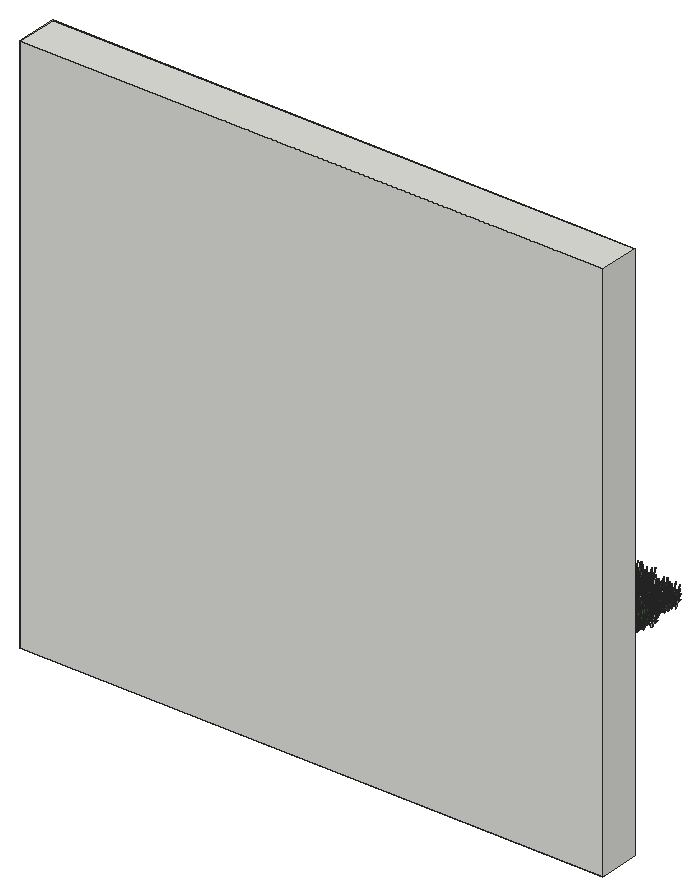
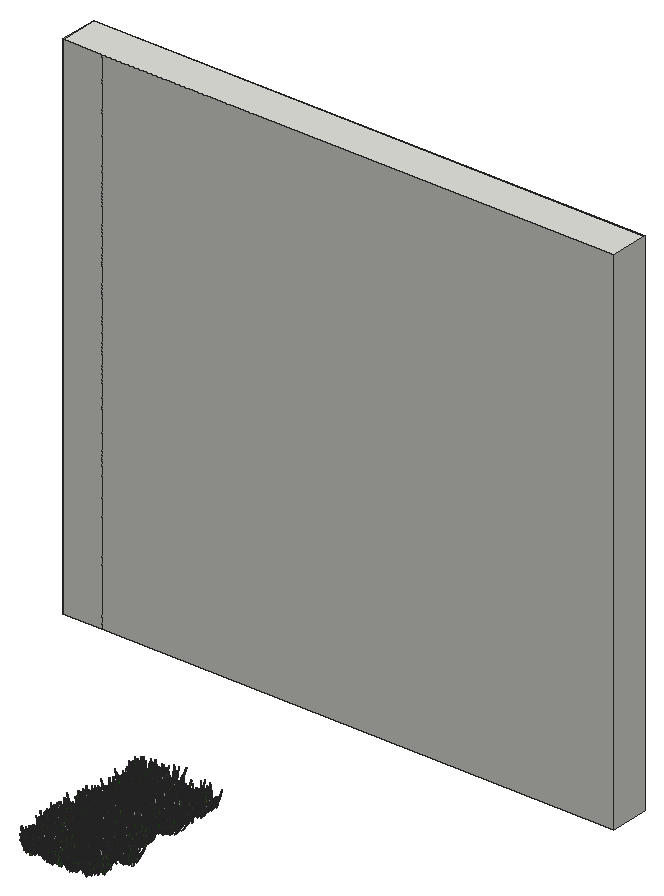
# SketchUp Ruby script. Lengths in inches.
U = 1.inch
M = Sketchup.active_model
def pt(a) = Geom::Point3d.new(a.map { |v| v * U })
def face(e, loops, mat)
  f = e.add_face(loops[0].map { |a| pt(a) })
  loops[1..].each { |l| e.add_face(l.map { |a| pt(a) }).erase! }
  f.material = f.back_material = mat if mat
  f
end
# faces: each face lists its corners as indices into pts; further lists are holes
def faces(e, pts, list, mat = nil) = list.each { |f| face(e, (f[0].is_a?(Array) ? f : [f]).map { |l| l.map { |i| pts[i] } }, mat) }
# xy, xz, yz: faces in a plane at the given z, y or x. An outline is a flat list of corners, or four numbers for a rectangle; further outlines are holes
def ring(l) = l.size == 4 ? [[l[0], l[1]], [l[2], l[1]], [l[2], l[3]], [l[0], l[3]]] : l.each_slice(2).to_a
def flat(e, list, mat, &to3) = list.each { |f| face(e, (f[0].is_a?(Array) ? f : [f]).map { |l| ring(l).map { |u, v| to3.(u, v) } }, mat) }
def xy(e, z, list, mat = nil) = flat(e, list, mat) { |x, y| [x, y, z] }
def xz(e, y, list, mat = nil) = flat(e, list, mat) { |x, z| [x, y, z] }
def yz(e, x, list, mat = nil) = flat(e, list, mat) { |y, z| [x, y, z] }
def lines(e, pts, list) = list.each { |a, b| e.add_line(pt(pts[a]), pt(pts[b])) }
# prism: a flat outline (further loops are holes) pulled along v
def prism(e, loops, v, mat = nil)
  f = face(e, loops, mat); d = Geom::Vector3d.new(v.map { |x| x * U })
  f.pushpull(f.normal.samedirection?(d) ? d.length : -d.length)
end
def box(e, o, s, mat = nil) = prism(e, [[o, [o[0] + s[0], o[1], o[2]], [o[0] + s[0], o[1] + s[1], o[2]], [o[0], o[1] + s[1], o[2]]]], [0, 0, s[2]], mat)
def at(x, y, z, deg = 0) = Geom::Transformation.translation(pt([x, y, z])) * Geom::Transformation.rotation(ORIGIN, Z_AXIS, deg.degrees)
def axes(o, x, y, z) = Geom::Transformation.new([*x, 0, *y, 0, *z, 0, *pt(o).to_a, 1])
def part(name) = M.definitions.add(name)
# library, detail: a bought-in or finely detailed component or shape, given as its bounding box
def library(name, o, s) = part(name).tap { |d| box(d.entities, o, s) }
def detail(e, o, s) = box(e.add_group.entities, o, s)
def put(e, d, t, mat = nil) = e.add_instance(d, t).tap { |i| i.material = mat if mat }
def group(e, t, mat = nil) = e.add_group.tap { |g| g.transformation = t; g.material = mat if mat }.entities
root = M.entities
M.materials.add("Material1").color = [58, 110, 58]
M.materials.add("Material10").color = [48, 100, 38]
M.materials.add("Material3").color = [68, 110, 58]
M.materials.add("Material4").color = [48, 90, 38]
M.materials.add("Material5").color = [68, 110, 48]
M.materials.add("Material6").color = [48, 90, 48]
M.materials.add("Material8").color = [58, 90, 38]
M.materials.add("Material9").color = [68, 100, 58]
c1 = part("grass00")
p = [[-0.6875,0.15,0],[-0.56,0.08,5.52],[-0.04,0.03,2.76],[0.48,-0.02,0],[0.35,-0.02,5.52],[-0.1,-0.14,5.52],
  [-0.12,0.65,8.37],[-0.42,0.65,8.37]]
faces(c1.entities,p,[[0,1,2,3],[3,2,4],[1,5,2],[5,4,2],[1,6,5],[4,5,6],[7,6,1]])
c2 = part("Group16\#1")
put(c2.entities,c1,axes([1.44,-0.61,-0.01],[0.05352,0.12609,0],[-0.10704,0.04543,0.07239],[0.06664,-0.02828,0.11628]),"Material6")
put(c2.entities,c1,axes([0.76,-0.15,-0.01],[0.04676,0.24062,0],[-0.23162,0.04501,0.06642],[0.0652,-0.01267,0.23595]),"Material3")
put(c2.entities,c1,axes([0.79,0.01,-0.01],[-0.00606,0.34651,0],[-0.34381,-0.00602,0.0432],[0.04319,0.00076,0.34386]))
put(c2.entities,c1,axes([1,0.23,-0.01],[-0.07192,0.31144,0],[-0.28722,-0.06632,0.1236],[0.12043,0.02781,0.29478]),"Material5")
put(c2.entities,c1,axes([1.66,0.77,-0.01],[-0.13828,0.29651,0],[-0.21551,-0.1005,0.22471],[0.20365,0.09498,0.23779]),"Material10")
put(c2.entities,c1,axes([0.6875,0.52,-0.01],[-0.18126,0.24051,0],[-0.22746,-0.17142,0.09788],[0.07817,0.05891,0.28481]),"Material5")
put(c2.entities,c1,axes([0.68,0.78,-0.01],[-0.215,0.18688,0],[-0.12385,-0.14248,0.21334],[0.13995,0.16101,0.18878]),"Material3")
put(c2.entities,c1,axes([0.56,1,-0.01],[-0.13756,0.07624,0],[-0.06159,-0.11112,0.0927],[0.04494,0.08108,0.12705]),"Material5")
put(c2.entities,c1,axes([0.2,0.64,-0.01],[-0.23729,0.07254,0],[-0.05711,-0.18681,0.153],[0.04473,0.14632,0.19535]),"Material10")
put(c2.entities,c1,axes([0.0625,0.72,-0.01],[-0.28874,0.02525,0],[-0.02179,-0.24916,0.14647],[0.01276,0.14591,0.25012]),"Material3")
put(c2.entities,c1,axes([-0.08,0.62,-0.01],[-0.34089,-0.04187,0],[0.03255,-0.26504,0.216],[-0.02633,0.21439,0.26703]),"Material10")
put(c2.entities,c1,axes([-0.34,0.98,-0.01],[-0.14314,-0.0493,0],[0.04397,-0.12769,0.06843],[-0.02228,0.0647,0.13505]),"Material10")
put(c2.entities,c1,axes([-0.87,1.45,-0.01],[-0.23488,-0.14114,0],[0.13761,-0.22901,0.06087],[-0.03135,0.05217,0.26717]))
put(c2.entities,c1,axes([-0.72,0.77,-0.01],[-0.14208,-0.13251,0],[0.07209,-0.0773,0.16301],[-0.11118,0.11922,0.1057]),"Material10")
put(c2.entities,c1,axes([-0.62,0.43,-0.01],[-0.14845,-0.21203,0],[0.18654,-0.13061,0.12304],[-0.10079,0.07057,0.22772]),"Material3")
put(c2.entities,c1,axes([-0.68,0.29,-0.01],[-0.13639,-0.32136,0],[0.31723,-0.13464,0.05579],[-0.05136,0.0218,0.34462]),"Material4")
put(c2.entities,c1,axes([-0.64,0.125,-0.01],[-0.0458,-0.23569,0],[0.22124,-0.043,0.08276],[-0.08124,0.01579,0.22538]),"Material1")
put(c2.entities,c1,axes([-1.6,-0.03,-0.01],[0.00576,-0.32897,0],[0.27526,0.00482,0.18018],[-0.18015,-0.00315,0.2753]),"Material5")
put(c2.entities,c1,axes([-1.36,-0.31,-0.01],[0.05718,-0.24765,0],[0.18172,0.04196,0.17267],[-0.16825,-0.03885,0.1865]),"Material10")
put(c2.entities,c1,axes([-1.54,-0.72,-0.01],[0.06537,-0.14017,0],[0.13555,0.06321,0.03939],[-0.0357,-0.01665,0.14956]))
put(c2.entities,c1,axes([-1.19,-0.9,-0.01],[0.09597,-0.12735,0],[0.11214,0.08451,0.07557],[-0.06035,-0.04548,0.14042]),"Material9")
put(c2.entities,c1,axes([-0.47,-0.54,-0.01],[0.11588,-0.10072,0],[0.0618,0.0711,0.12124],[-0.07953,-0.0915,0.0942]))
put(c2.entities,c1,axes([-0.47,-0.84,-0.01],[0.11927,-0.0661,0],[0.06603,0.11913,0.00646],[-0.00313,-0.00565,0.13621]),"Material5")
put(c2.entities,c1,axes([-0.38,-1.24,-0.01],[0.28037,-0.08571,0],[0.0618,0.20215,0.20315],[-0.05939,-0.19428,0.21139]),"Material9")
put(c2.entities,c1,axes([-0.06,-0.66,-0.01],[0.22719,-0.01987,0],[0.01247,0.14255,0.17758],[-0.01547,-0.17691,0.1431]),"Material8")
put(c2.entities,c1,axes([0.11,-0.89,-0.01],[0.14882,0.01828,0],[-0.01058,0.08611,0.12229],[0.01491,-0.12138,0.08676]),"Material6")
put(c2.entities,c1,axes([0.25,-0.72,-0.01],[0.20481,0.07053,0],[-0.06206,0.18022,0.10291],[0.03351,-0.0973,0.1906]),"Material6")
put(c2.entities,c1,axes([0.85,-1.42,-0.01],[0.16481,0.09904,0],[-0.09472,0.15762,0.05616],[0.02893,-0.04814,0.18389]),"Material5")
put(c2.entities,c1,axes([1.01,-1.09,-0.01],[0.21858,0.20385,0],[-0.17495,0.1876,0.15339],[0.10462,-0.11218,0.25652]),"Material10")
put(c2.entities,c1,axes([1.01,-0.71,-0.01],[0.08733,0.12473,0],[-0.06445,0.04512,0.13037],[0.1068,-0.07477,0.07867]),"Material6")
c3 = part("Group15\#1")
put(c3.entities,c2,at(0,0,0))
c4 = part("3darcstudiotree_grass00\#1")
put(c4.entities,c3,at(0,0,0))
put(root,c4,axes([280.14,122.01,0.25],[0.96649,0.69,0],[-0.71558,0.6905,-0.04839],[-0.04247,0.04099,1.47711]))
put(root,c4,axes([280.98,108.43,0.25],[-0.66676,-0.67151,0],[0.72285,-0.49444,-0.03867],[0.0477,-0.03263,1.49724]))
put(root,c4,axes([281.09,99.91,0.25],[-0.806,-0.35525,0],[0.5393,-0.84292,-0.05452],[0.03122,-0.0488,1.404]))
put(root,c4,axes([281.11,97.14,0.25],[0.1532,-1.04407,0],[1.04107,0.10524,-0.0324],[0.04538,0.00459,1.47946]))
put(root,c4,axes([281.3,104.07,0.25],[-0.11859,-0.98397,0],[1.04274,-0.08657,-0.05423],[0.08746,-0.00726,1.69842]))
put(root,c4,axes([281.33,106.17,0.25],[-0.91725,0.50365,0],[-0.56826,-0.71295,-0.03289],[-0.02742,-0.03441,1.55622]))
put(root,c4,axes([281.53,109.2,0.25],[-0.76435,-0.59481,0],[0.61932,-0.54826,-0.04465],[0.05797,-0.05132,1.71883]))
put(root,c4,axes([281.74,100.72,0.25],[-0.61176,-0.56382,0],[0.75936,-0.56761,-0.04825],[0.06504,-0.04861,1.85346]))
put(root,c4,axes([281.89,127.21,0.25],[-0.44538,0.78051,0],[-1.01343,-0.39838,-0.05633],[-0.08545,-0.03359,1.88219]))
put(root,c4,axes([282.54,120.57,0.25],[0.24659,-0.81567,0],[1.24028,0.2583,-0.03647],[0.03753,0.00782,1.35653]))
put(root,c4,axes([282.49,113.52,0.25],[0.32185,-0.85158,0],[0.94359,0.24568,-0.02865],[0.04831,0.01258,1.74795]))
put(root,c4,axes([282.39,104.88,0.25],[0.64389,-0.79793,0],[0.85629,0.47602,-0.05113],[0.06464,0.03594,1.56833]))
put(root,c4,axes([282.72,108.55,0.25],[-0.90263,-0.3415,0],[0.38015,-0.6922,-0.0331],[0.02315,-0.04215,1.54531]))
put(root,c4,axes([282.41,106.7,0.25],[0.73285,0.722,0],[-0.72451,0.50662,-0.04423],[-0.04928,0.03446,1.38013]))
put(root,c4,axes([282.86,114.61,0.25],[-0.198,-0.93495,0],[1.04135,-0.15193,-0.04893],[0.07876,-0.01149,1.72817]))
put(root,c4,axes([282.61,122.33,0.25],[1.14207,-0.102,0],[0.13761,1.06147,-0.03237],[0.00412,0.03176,1.52951]))
put(root,c4,axes([283.03,103.375,0.25],[-1.16606,-0.38849,0],[0.34532,-0.71405,-0.04034],[0.02573,-0.05319,1.58691]))
g1 = group(root,at(186.47,48,0))
prism(g1,[[[151.5,9,0],[160.5,9,0],[160.5,0,0],[32.14,0,0],[32.14,9,0]]],[0,0,120])
put(root,c4,axes([282.7,129.27,0.25],[0.32926,0.73623,0],[-0.88152,0.27159,-0.04291],[-0.06174,0.01902,1.44315]))
put(root,c4,axes([282.91,125.12,0.25],[0.71198,-0.69558,0],[0.87959,0.62024,-0.02612],[0.03242,0.02286,1.8801]))
put(root,c4,axes([282.76,98.67,0.25],[-0.09062,0.98179,0],[-1.0736,-0.06826,-0.03234],[-0.05691,-0.00362,1.90052]))
put(root,c4,axes([282.67,116.89,0.25],[1.06044,0.60949,0],[-0.58603,0.70241,-0.05103],[-0.04763,0.05709,1.6877]))
put(root,c4,axes([283.35,110.84,0.25],[0.39396,-0.77569,0],[0.86907,0.30407,-0.03331],[0.04938,0.01728,1.51731]))
put(root,c4,axes([283.38,126.24,0.25],[0.16763,0.79034,0],[-1.21049,0.17687,-0.06022],[-0.08603,0.01257,1.78296]))
put(root,c4,axes([283.39,111.61,0.25],[0.53853,0.6124,0],[-0.87052,0.52736,-0.05552],[-0.05804,0.03516,1.39481]))
put(root,c4,axes([284.24,112.93,0.25],[-1.23083,0.12452,0],[-0.1215,-0.82732,-0.03065],[-0.0073,-0.04972,1.97713]))
put(root,c4,axes([284.36,124.27,0.25],[-0.86307,-0.26422,0],[0.42976,-0.96707,-0.02933],[0.01407,-0.03166,1.72129]))
put(root,c4,axes([284.12,100.69,0.25],[1.06091,-0.11039,0],[0.1522,1.0077,-0.03701],[0.00751,0.0497,1.99511]))
put(root,c4,axes([284.06,116.32,0.25],[1.09581,0.45799,0],[-0.53398,0.88015,-0.03278],[-0.02339,0.03856,1.8841]))
put(root,c4,axes([284.42,112.27,0.25],[0.45131,-0.77831,0],[1.15874,0.46288,-0.06017],[0.07334,0.0293,1.73941]))
put(root,c4,axes([284.17,122.08,0.25],[0.99888,0.1401,0],[-0.16713,0.82088,-0.04218],[-0.013,0.06385,1.85529]))
put(root,c4,axes([284.58,104.35,0.25],[-0.30186,-0.76108,0],[1.1493,-0.31403,-0.05688],[0.08145,-0.02225,1.82396]))
put(root,c4,axes([284.15,109.83,0.25],[1.15021,0.22516,0],[-0.24972,0.8788,-0.02883],[-0.0112,0.03942,1.84132]))
put(root,c4,axes([284.75,123.19,0.25],[-0.72312,-0.52329,0],[0.69977,-0.66616,-0.03875],[0.0408,-0.03885,1.70607]))
put(root,c4,axes([284.55,108.29,0.25],[0.68383,-0.50222,0],[0.78836,0.7395,-0.04815],[0.0527,0.04943,1.9649]))
put(root,c4,axes([284.48,125.64,0.25],[0.97755,0.3703,0],[-0.38502,0.7002,-0.03533],[-0.0295,0.05366,1.86502]))
put(root,c4,axes([284.8125,119.35,0.25],[-0.12292,0.83093,0],[-1.10355,-0.11246,-0.03564],[-0.05441,-0.00554,1.71014]))
put(root,c4,axes([284.75,118.61,0.25],[0.6999,0.62264,0],[-0.94819,0.73425,-0.03325],[-0.02999,0.02322,1.59934]))
put(root,c4,axes([285.35,116.27,0.25],[0.07977,-1.03792,0],[1.09466,0.05796,-0.05413],[0.06849,0.00363,1.39055]))
put(root,c4,axes([285.41,107.9,0.25],[0.16518,-1.06009,0],[1.27092,0.13643,-0.05291],[0.05462,0.00586,1.33374]))
put(root,c4,axes([285.51,114.64,0.25],[0.73988,-0.77354,0],[1.00505,0.66225,-0.06314],[0.05015,0.03304,1.30132]))
put(root,c4,axes([285.9,129.72,0.25],[-0.53978,-0.75827,0],[1.09521,-0.53709,-0.05519],[0.06778,-0.03324,1.81465]))
put(root,c4,axes([285.54,104.98,0.25],[0.1922,0.82569,0],[-0.98101,0.15731,-0.03785],[-0.05301,0.0085,1.42505]))
put(root,c4,axes([286.08,107,0.25],[-1.10209,-0.52404,0],[0.57256,-0.82953,-0.04075],[0.02735,-0.03962,1.55523]))
put(root,c4,axes([286.09,123.16,0.25],[-0.23218,-0.75967,0],[1.05774,-0.22271,-0.05601],[0.08968,-0.01888,1.80254]))
put(root,c4,axes([286.37,121.05,0.25],[-1.03868,-0.27875,0],[0.37896,-0.97279,-0.04655],[0.01837,-0.04716,1.58019]))
put(root,c4,axes([286.02,100.5625,0.25],[0.98254,-0.25265,0],[0.27656,0.74092,-0.04073],[0.01854,0.04967,1.43775]))
put(root,c4,axes([286.03,99.6,0.25],[0.41986,0.75322,0],[-1.13167,0.43457,-0.03574],[-0.04976,0.01911,1.91331]))
put(root,c4,axes([286.16,124.78,0.25],[1.16546,0.46684,0],[-0.47037,0.80896,-0.05424],[-0.02973,0.05113,1.36476]))
put(root,c4,axes([286.47,111.74,0.25],[0.34768,-0.86387,0],[0.85624,0.2374,-0.03453],[0.0639,0.01772,1.76116]))
put(root,c4,axes([286.92,106.86,0.25],[-1.17297,-0.02067,0],[0.02407,-0.94108,-0.04949],[0.00177,-0.06917,1.9102]))
put(root,c4,axes([287.3,120.81,0.25],[-0.61007,-0.79395,0],[0.95148,-0.50366,-0.04256],[0.04955,-0.02623,1.55835]))
put(root,c4,axes([286.97,127.42,0.25],[0.91396,-0.02464,0],[0.04119,1.05258,-0.05593],[0.0023,0.05867,1.60461]))
put(root,c4,axes([287.07,117.22,0.25],[1.02052,0.55135,0],[-0.53482,0.68197,-0.02904],[-0.02865,0.03654,1.7729]))
put(root,c4,axes([287.17,108.65,0.25],[0.83736,0.33838,0],[-0.55915,0.95321,-0.05845],[-0.03084,0.05257,1.53958]))
put(root,c4,axes([287.625,103.1,0.25],[-1.22566,0.31592,0],[-0.30293,-0.80966,-0.03919],[-0.01931,-0.05162,1.69748]))
put(root,c4,axes([287.47,99.875,0.25],[0.97887,-0.22338,0],[0.25967,0.78389,-0.03828],[0.01628,0.04916,1.57185]))
put(root,c4,axes([287.42,115.04,0.25],[1.01452,0.22805,0],[-0.26327,0.80685,-0.0432],[-0.01701,0.05214,1.51727]))
put(root,c4,axes([287.625,100.98,0.25],[-0.59004,0.75476,0],[-0.98006,-0.52782,-0.05659],[-0.05684,-0.03061,1.39892]))
put(root,c4,axes([287.92,112.15,0.25],[0.76894,-0.45763,0],[0.64505,0.74668,-0.04704],[0.04225,0.0489,1.70604]))
put(root,c4,axes([287.92,109.35,0.25],[1.18056,0.12682,0],[-0.16494,1.05779,-0.04718],[-0.00694,0.0445,1.4726]))
put(root,c4,axes([287.99,102.05,0.25],[0.2316,1.00827,0],[-0.94622,0.14973,-0.03349],[-0.05489,0.00869,1.60736]))
put(root,c4,axes([287.99,105.91,0.25],[1.03219,0.4525,0],[-0.48048,0.75505,-0.05015],[-0.04152,0.06525,1.82381]))
put(root,c4,axes([288.62,106.05,0.25],[0.66048,-0.81262,0],[0.83349,0.46669,-0.04469],[0.06734,0.0377,1.8275]))
put(root,c4,axes([288.92,116.05,0.25],[-0.79781,-0.64301,0],[0.72834,-0.62256,-0.03796],[0.04001,-0.0342,1.58175]))
put(root,c4,axes([288.49,124.47,0.25],[-0.01446,0.75216,0],[-1.24873,-0.01654,-0.04794],[-0.0632,-0.00084,1.64652]))
put(root,c4,axes([288.79,117.9,0.25],[0.43992,-0.87485,0],[0.97647,0.33827,-0.05171],[0.0741,0.02567,1.64301]))
put(root,c4,axes([288.66,126.91,0.25],[0.12832,0.79022,0],[-1.17061,0.13096,-0.05207],[-0.07812,0.00874,1.7882]))
put(root,c4,axes([289.1,102.97,0.25],[-0.8223,-0.75997,0],[0.923,-0.68801,-0.05274],[0.06284,-0.04684,1.98669]))
put(root,c4,axes([288.86,123.09,0.25],[1.11111,0.21953,0],[-0.27842,0.97075,-0.06215],[-0.01955,0.06815,1.63292]))
put(root,c4,axes([289.36,119.46,0.25],[-0.90252,-0.41614,0],[0.59502,-0.889,-0.02959],[0.01936,-0.02892,1.65043]))
put(root,c4,axes([288.92,122.25,0.25],[0.40373,0.79991,0],[-1.04976,0.365,-0.03717],[-0.04874,0.01695,1.61797]))
put(root,c4,axes([288.93,110.84,0.25],[0.79847,0.56552,0],[-0.69028,0.67142,-0.03219],[-0.03713,0.03611,1.88986]))
put(root,c4,axes([289.32,107.31,0.25],[1.12258,-0.30459,0],[0.34364,0.87251,-0.04269],[0.02321,0.05894,1.93529]))
put(root,c4,axes([289.49,104.47,0.25],[0.7553,-0.61251,0],[0.83696,0.71099,-0.03867],[0.0393,0.03338,1.7417]))
put(root,c4,axes([290.03,115.75,0.25],[-1.07836,-0.58735,0],[0.50923,-0.64407,-0.04657],[0.05066,-0.06408,1.84036]))
put(root,c4,axes([289.92,119.61,0.25],[0.69922,-0.64094,0],[0.77633,0.58344,-0.04299],[0.04858,0.03651,1.59659]))
put(root,c4,axes([290.17,97.35,0.25],[-0.83056,-0.81172,0],[0.84588,-0.59626,-0.05304],[0.07118,-0.05018,1.95407]))
put(root,c4,axes([289.98,122.11,0.25],[-0.57712,0.80927,0],[-0.96213,-0.47267,-0.03668],[-0.05591,-0.02747,1.98009]))
put(root,c4,axes([290.04,129.82,0.25],[-0.4755,0.85123,0],[-1.1316,-0.43547,-0.04346],[-0.05893,-0.02268,1.86413]))
put(root,c4,axes([290.375,113.57,0.25],[-1.24305,0.08795,0],[-0.08349,-0.8129,-0.04632],[-0.00759,-0.07395,1.89764]))
put(root,c4,axes([290.38,118.09,0.25],[-0.3366,0.79048,0],[-0.85568,-0.25101,-0.03966],[-0.05713,-0.01676,1.38647]))
put(root,c4,axes([290.51,111.18,0.25],[-0.95842,0.70962,0],[-0.69168,-0.64356,-0.04505],[-0.0402,-0.0374,1.39266]))
put(root,c4,axes([290.77,116.66,0.25],[-0.37206,-0.80051,0],[1.04801,-0.33556,-0.03571],[0.05709,-0.01828,1.92492]))
put(root,c4,axes([290.39,128.52,0.25],[0.53635,0.81697,0],[-0.91633,0.41443,-0.025],[-0.04192,0.01896,1.99255]))
put(root,c4,axes([290.84,112.06,0.25],[-1.12484,0.02949,0],[-0.03445,-0.90524,-0.03959],[-0.00189,-0.04972,1.65212]))
put(root,c4,axes([290.43,106.58,0.25],[0.762,0.81603,0],[-0.98717,0.63503,-0.03267],[-0.04011,0.0258,1.93988]))
put(root,c4,axes([290.47,126.36,0.25],[0.38959,0.87785,0],[-1.14834,0.35109,-0.04046],[-0.04842,0.0148,1.56076]))
put(root,c4,axes([290.5,104.11,0.25],[0.00735,0.80444,0],[-1.27856,0.00805,-0.03677],[-0.03983,0.00025,1.38481]))
put(root,c4,axes([290.98,99.38,0.25],[-1.06799,-0.08228,0],[0.11727,-1.04872,-0.06502],[0.00676,-0.06047,1.42798]))
put(root,c4,axes([291,103.25,0.25],[0.37646,-0.94503,0],[1.15519,0.31701,-0.04027],[0.05381,0.01477,1.71232]))
put(root,c4,axes([291.6,110.66,0.25],[-0.25978,-0.80409,0],[1.2428,-0.2766,-0.04199],[0.05612,-0.01249,1.7807]))
put(root,c4,axes([291.7,114.34,0.25],[-0.702,-0.60475,0],[0.80009,-0.63981,-0.03217],[0.03306,-0.02644,1.58546]))
put(root,c4,axes([291.61,103.15,0.25],[-1.15974,0.17681,0],[-0.23333,-1.05436,-0.05609],[-0.01523,-0.06884,1.94158]))
put(root,c4,axes([291.68,108.77,0.25],[-1.05103,-0.44112,0],[0.40767,-0.66914,-0.0255],[0.02475,-0.04062,1.94297]))
put(root,c4,axes([291.6,129.58,0.25],[-0.88188,0.19198,0],[-0.31522,-0.99749,-0.03948],[-0.01275,-0.04035,1.58152]))
put(root,c4,axes([291.52,101.04,0.25],[0.03817,0.87199,0],[-0.96597,0.02913,-0.04285],[-0.08096,0.00244,1.82733]))
put(root,c4,axes([291.57,123.71,0.25],[0.92789,-0.22475,0],[0.34756,0.98849,-0.04654],[0.01412,0.04015,1.34343]))
put(root,c4,axes([291.5,128.36,0.25],[0.99429,0.37074,0],[-0.40917,0.75597,-0.04301],[-0.02965,0.05478,1.6797]))
put(root,c4,axes([291.66,109.25,0.25],[0.96625,-0.29228,0],[0.40926,0.93206,-0.06136],[0.03176,0.07234,1.80687]))
put(root,c4,axes([292.2,99.92,0.25],[-1.17693,0.29826,0],[-0.36809,-1.0006,-0.03433],[-0.01076,-0.02926,1.35329]))
put(root,c4,axes([292.15,105.75,0.25],[-0.17663,0.73999,0],[-1.12217,-0.18452,-0.03573],[-0.05134,-0.00844,1.67549]))
put(root,c4,axes([292.33,111.77,0.25],[-0.24663,0.96758,0],[-1.21778,-0.21384,-0.05558],[-0.06952,-0.01221,1.59125]))
put(root,c4,axes([293,108.58,0.25],[-0.43903,-0.74591,0],[0.90583,-0.36729,-0.0349],[0.05733,-0.02325,1.84302]))
put(root,c4,axes([293.16,116.25,0.25],[-1.05707,-0.00531,0],[0.00764,-1.04694,-0.0591],[0.00043,-0.05923,1.52309]))
put(root,c4,axes([293.22,113.8,0.25],[-1.17737,-0.08134,0],[0.09201,-0.91752,-0.036],[0.00525,-0.05238,1.9513]))
put(root,c4,axes([293.1,120.42,0.25],[0.22942,-0.80247,0],[0.87812,0.17294,-0.04624],[0.09726,0.01916,1.95114]))
put(root,c4,axes([293.1,126.04,0.25],[-0.55637,0.80922,0],[-0.80968,-0.3835,-0.04437],[-0.06055,-0.02868,1.46464]))
put(root,c4,axes([293.35,97.26,0.25],[0.33509,-0.89072,0],[1.18941,0.30825,-0.04262],[0.0593,0.01537,1.81655]))
put(root,c4,axes([293.36,104.52,0.25],[-0.67254,0.91689,0],[-0.85898,-0.43406,-0.03488],[-0.04061,-0.02052,1.37068]))
put(root,c4,axes([293.24,107.32,0.25],[0.92619,-0.10185,0],[0.12918,0.80925,-0.04905],[0.00971,0.06081,1.48186]))
put(root,c4,axes([293.41,99.89,0.25],[0.87821,-0.27516,0],[0.35278,0.77567,-0.04981],[0.0297,0.06529,1.68613]))
put(root,c4,axes([293.75,114.91,0.25],[-0.56452,-0.83255,0],[0.9394,-0.43881,-0.05229],[0.06965,-0.03253,1.64764]))
put(root,c4,axes([293.53,109.625,0.25],[-0.60052,0.95546,0],[-1.10338,-0.47774,-0.04188],[-0.0563,-0.02437,1.88687]))
put(root,c4,axes([293.36,122.25,0.25],[0.78993,0.53505,0],[-0.70019,0.71214,-0.03119],[-0.03391,0.03449,1.90467]))
put(root,c4,axes([293.67,128.55,0.25],[-0.50113,0.91608,0],[-0.83688,-0.31538,-0.0444],[-0.07161,-0.02699,1.62807]))
put(root,c4,axes([293.77,118.05,0.25],[-0.62087,0.78586,0],[-1.03493,-0.56328,-0.05216],[-0.04615,-0.02512,1.30947]))
put(root,c4,axes([293.77,119.28,0.25],[-0.50471,0.92883,0],[-1.16901,-0.43761,-0.03185],[-0.04122,-0.01543,1.82087]))
put(root,c4,axes([293.79,103.3,0.25],[0.56865,0.58347,0],[-0.72151,0.48442,-0.02717],[-0.04145,0.02783,1.82093]))
put(root,c4,axes([293.82,98.21,0.25],[0.94731,0.21958,0],[-0.24315,0.72265,-0.03829],[-0.01599,0.04753,1.40372]))
put(root,c4,axes([293.96,124.92,0.25],[1.08833,-0.17129,0],[0.24008,1.05081,-0.05959],[0.01345,0.05887,1.56123]))
put(root,c4,axes([294.57,98.01,0.25],[-0.98856,-0.22721,0],[0.32875,-0.98537,-0.02644],[0.01092,-0.03274,1.9068]))
put(root,c4,axes([294.76,121,0.25],[-1.06378,-0.45854,0],[0.55437,-0.88599,-0.03725],[0.0222,-0.03547,1.55507]))
put(root,c4,axes([294.55,128.33,0.25],[-0.74093,0.83806,0],[-0.99545,-0.60629,-0.06171],[-0.06944,-0.04229,1.72322]))
put(root,c4,axes([294.48,124.32,0.25],[0.46742,0.64787,0],[-0.79059,0.39294,-0.04808],[-0.08341,0.04146,1.86326]))
put(root,c4,axes([294.47,114.3125,0.25],[1.2015,-0.12231,0],[0.11788,0.79771,-0.03723],[0.00613,0.04149,1.30959]))
put(root,c4,axes([294.98,116.07,0.25],[-0.59629,-0.71141,0],[0.97299,-0.56183,-0.03629],[0.03633,-0.02098,1.44541]))
put(root,c4,axes([295.01,113.25,0.25],[-0.63803,-0.55932,0],[0.93956,-0.73835,-0.06171],[0.05652,-0.04442,1.63202]))
put(root,c4,axes([294.99,119.72,0.25],[-0.74714,0.45466,0],[-0.55607,-0.6295,-0.03589],[-0.04356,-0.04931,1.93035]))
put(root,c4,axes([294.98,117.41,0.25],[-0.41307,0.85802,0],[-0.98988,-0.32829,-0.0529],[-0.07297,-0.0242,1.58349]))
put(root,c4,axes([294.81,99.62,0.25],[1.25345,0.24308,0],[-0.21659,0.76943,-0.04207],[-0.01337,0.0475,1.32997]))
put(root,c4,axes([295.15,104.22,0.25],[-0.76344,0.78897,0],[-0.79052,-0.52697,-0.04358],[-0.05588,-0.03725,1.66757]))
put(root,c4,axes([294.96,111.9375,0.25],[0.98308,0.32304,0],[-0.38251,0.80192,-0.03237],[-0.01873,0.03927,1.63378]))
put(root,c4,axes([295.52,123.75,0.25],[-1.15457,-0.02689,0],[0.02641,-0.78117,-0.03959],[0.00231,-0.06847,1.96257]))
put(root,c4,axes([295.1,109.62,0.25],[1.12266,0.48288,0],[-0.58126,0.93097,-0.0509],[-0.02988,0.04786,1.61215]))
put(root,c4,axes([295.54,105.79,0.25],[0.84091,-0.32955,0],[0.43979,0.77307,-0.03456],[0.02389,0.04199,1.66747]))
put(root,c4,axes([295.57,126.78,0.25],[-0.20753,0.73084,0],[-0.89975,-0.17601,-0.04738],[-0.07204,-0.01409,1.4441]))
put(root,c4,axes([296,129.73,0.25],[-0.98261,0.10155,0],[-0.1134,-0.75589,-0.03309],[-0.00716,-0.04773,1.60704]))
put(root,c4,axes([296.01,97.1,0.25],[0.59431,-0.75291,0],[0.96844,0.52662,-0.04807],[0.05897,0.03206,1.69791]))
put(root,c4,axes([296.05,110.87,0.25],[0.68985,-0.67719,0],[0.83775,0.58792,-0.03628],[0.03764,0.02641,1.49031]))
put(root,c4,axes([296.28,123.13,0.25],[-0.46608,-0.832,0],[0.83606,-0.32265,-0.04244],[0.07949,-0.03068,1.90455]))
put(root,c4,axes([296.6,111.78,0.25],[-0.51956,-0.89208,0],[1.01347,-0.40663,-0.04214],[0.05256,-0.02109,1.55921]))
put(root,c4,axes([296.24,115.74,0.25],[-0.17363,0.82536,0],[-1.01711,-0.1474,-0.03794],[-0.05162,-0.00748,1.42617]))
put(root,c4,axes([296.39,101.7,0.25],[-0.51524,0.80419,0],[-0.85078,-0.37551,-0.04799],[-0.08762,-0.03867,1.99284]))
put(root,c4,axes([296.61,128.21,0.25],[0.05532,-0.99305,0],[1.16992,0.0449,-0.04434],[0.05856,0.00225,1.54852]))
put(root,c4,axes([296.61,119.73,0.25],[-0.62549,0.93187,0],[-1.04928,-0.48519,-0.0557],[-0.0628,-0.02904,1.55009]))
put(root,c4,axes([296.96,121.9,0.25],[-0.8786,-0.78973,0],[0.94499,-0.72426,-0.04946],[0.04193,-0.03214,1.48426]))
put(root,c4,axes([296.91,114.21,0.25],[-1.09931,-0.14052,0],[0.14882,-0.80208,-0.03709],[0.00974,-0.05249,1.68681]))
put(root,c4,axes([296.8125,113.22,0.25],[-0.85433,0.32747,0],[-0.49892,-0.89669,-0.05064],[-0.02624,-0.04715,1.47033]))
put(root,c4,axes([296.99,120.44,0.25],[0.53888,-0.61524,0],[0.84696,0.51105,-0.02782],[0.04065,0.02453,1.89124]))
put(root,c4,axes([296.85,109.875,0.25],[0.65312,0.54647,0],[-0.82088,0.67587,-0.03885],[-0.03791,0.03121,1.58937]))
put(root,c4,axes([296.99,117.49,0.25],[0.85152,0.26385,0],[-0.40716,0.90523,-0.03179],[-0.0169,0.03757,1.76952]))
